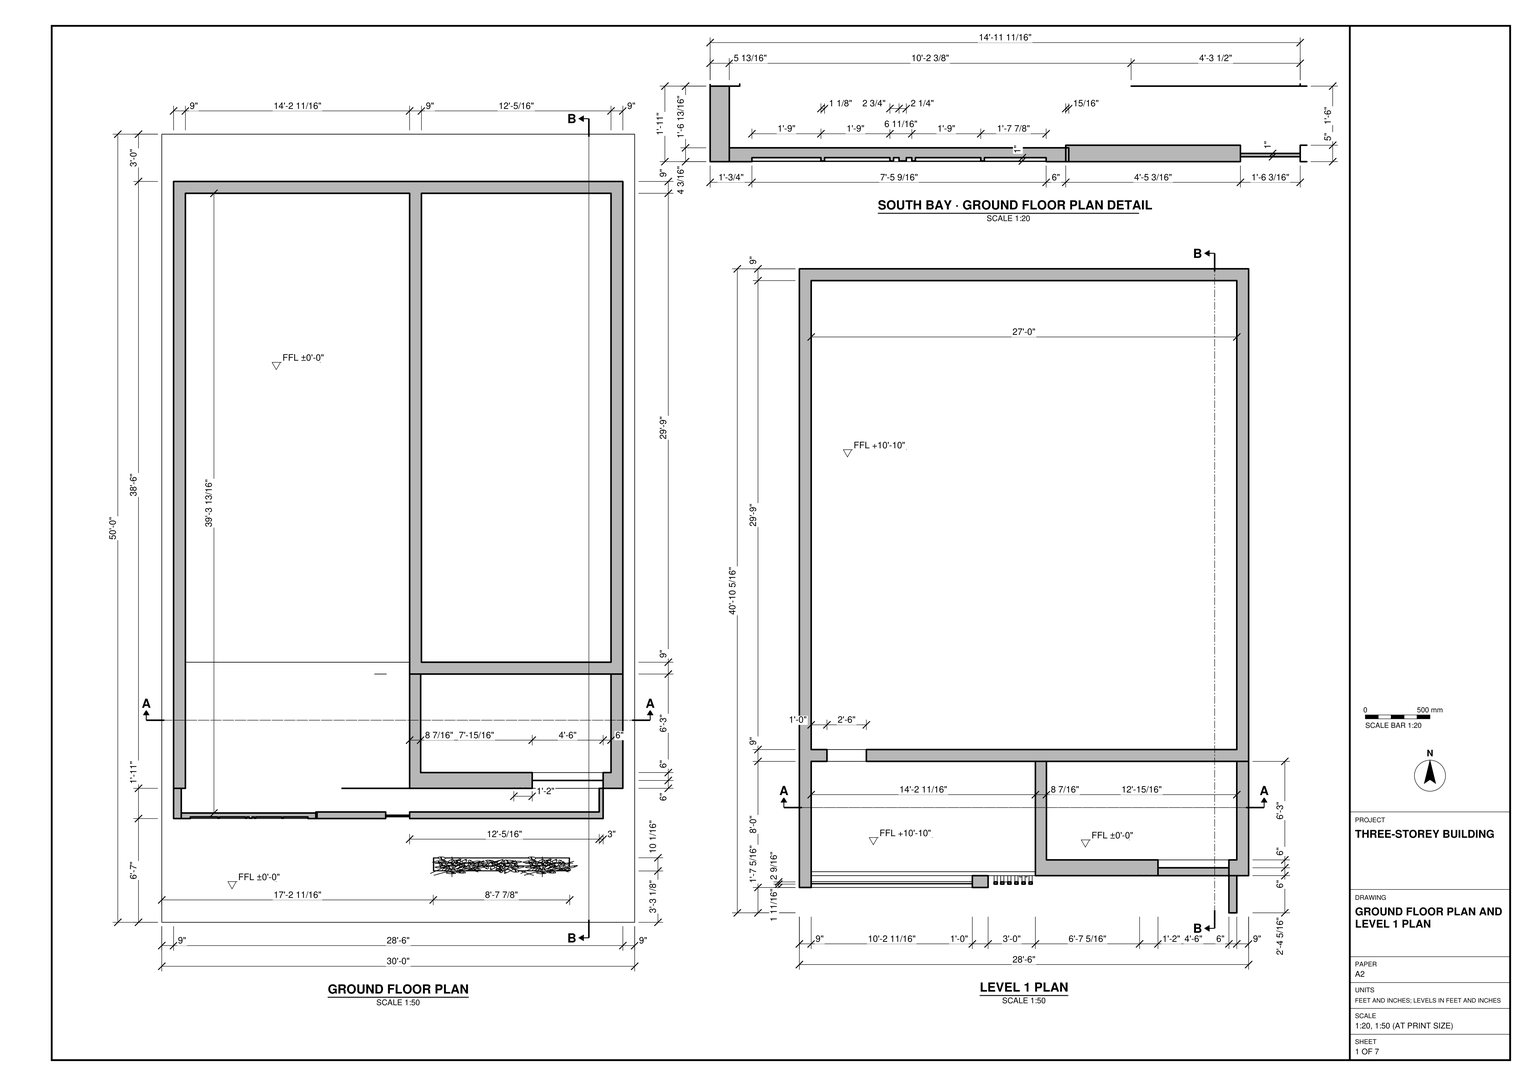
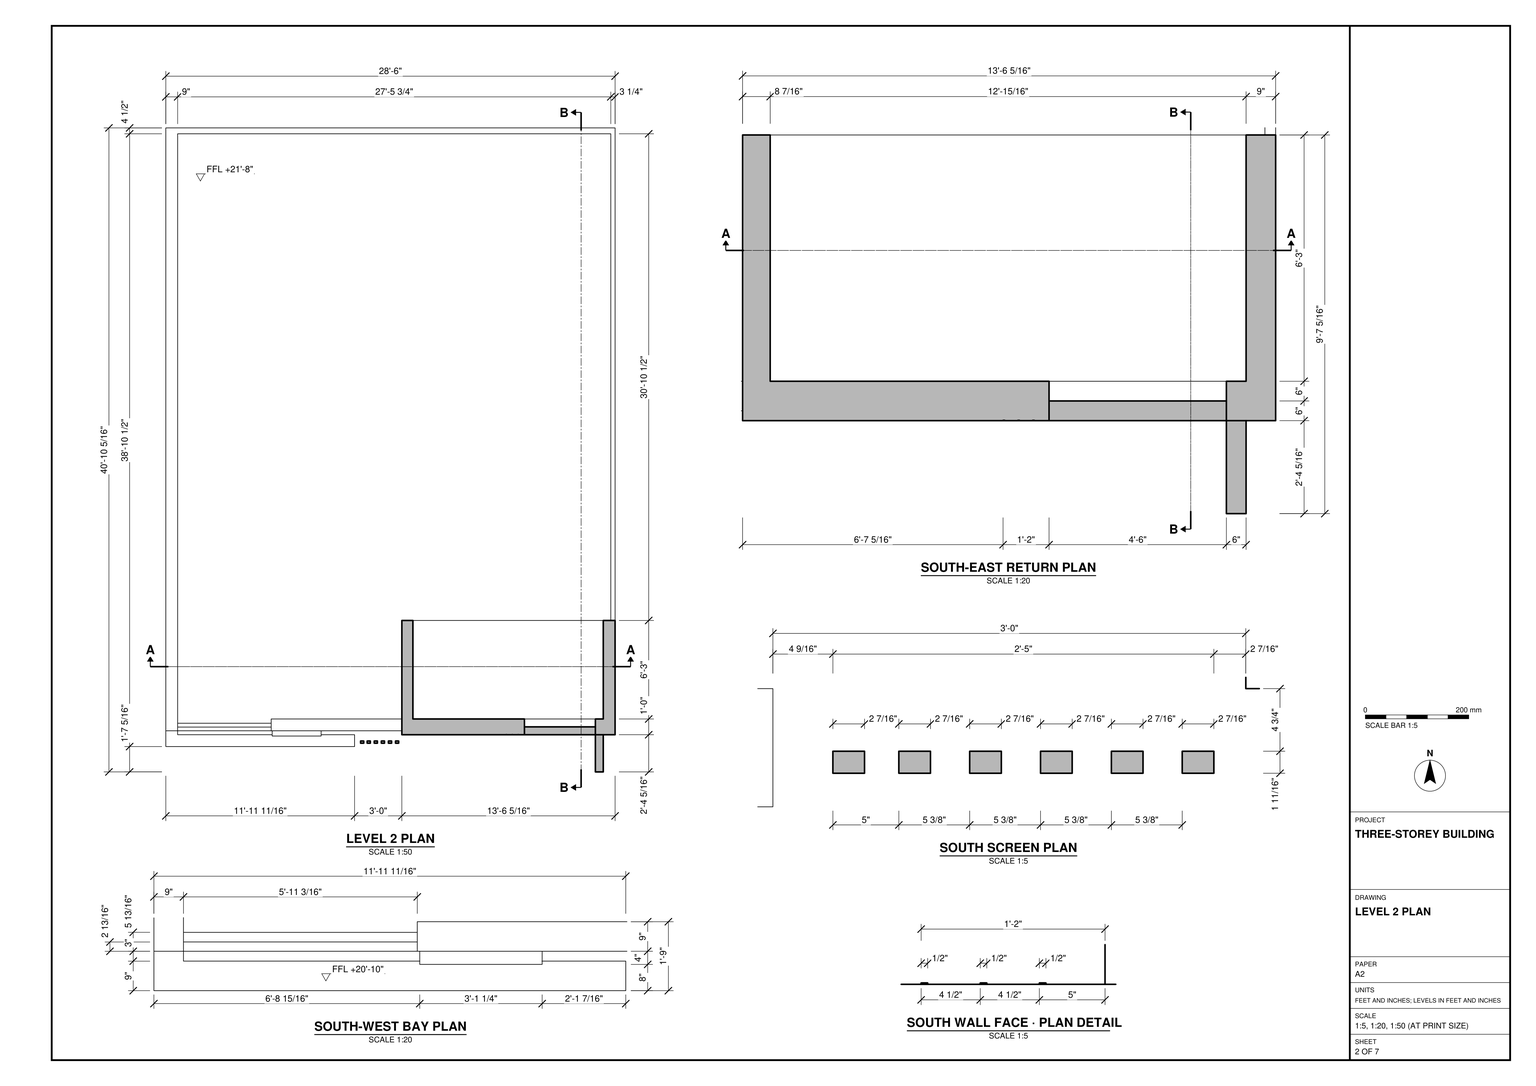
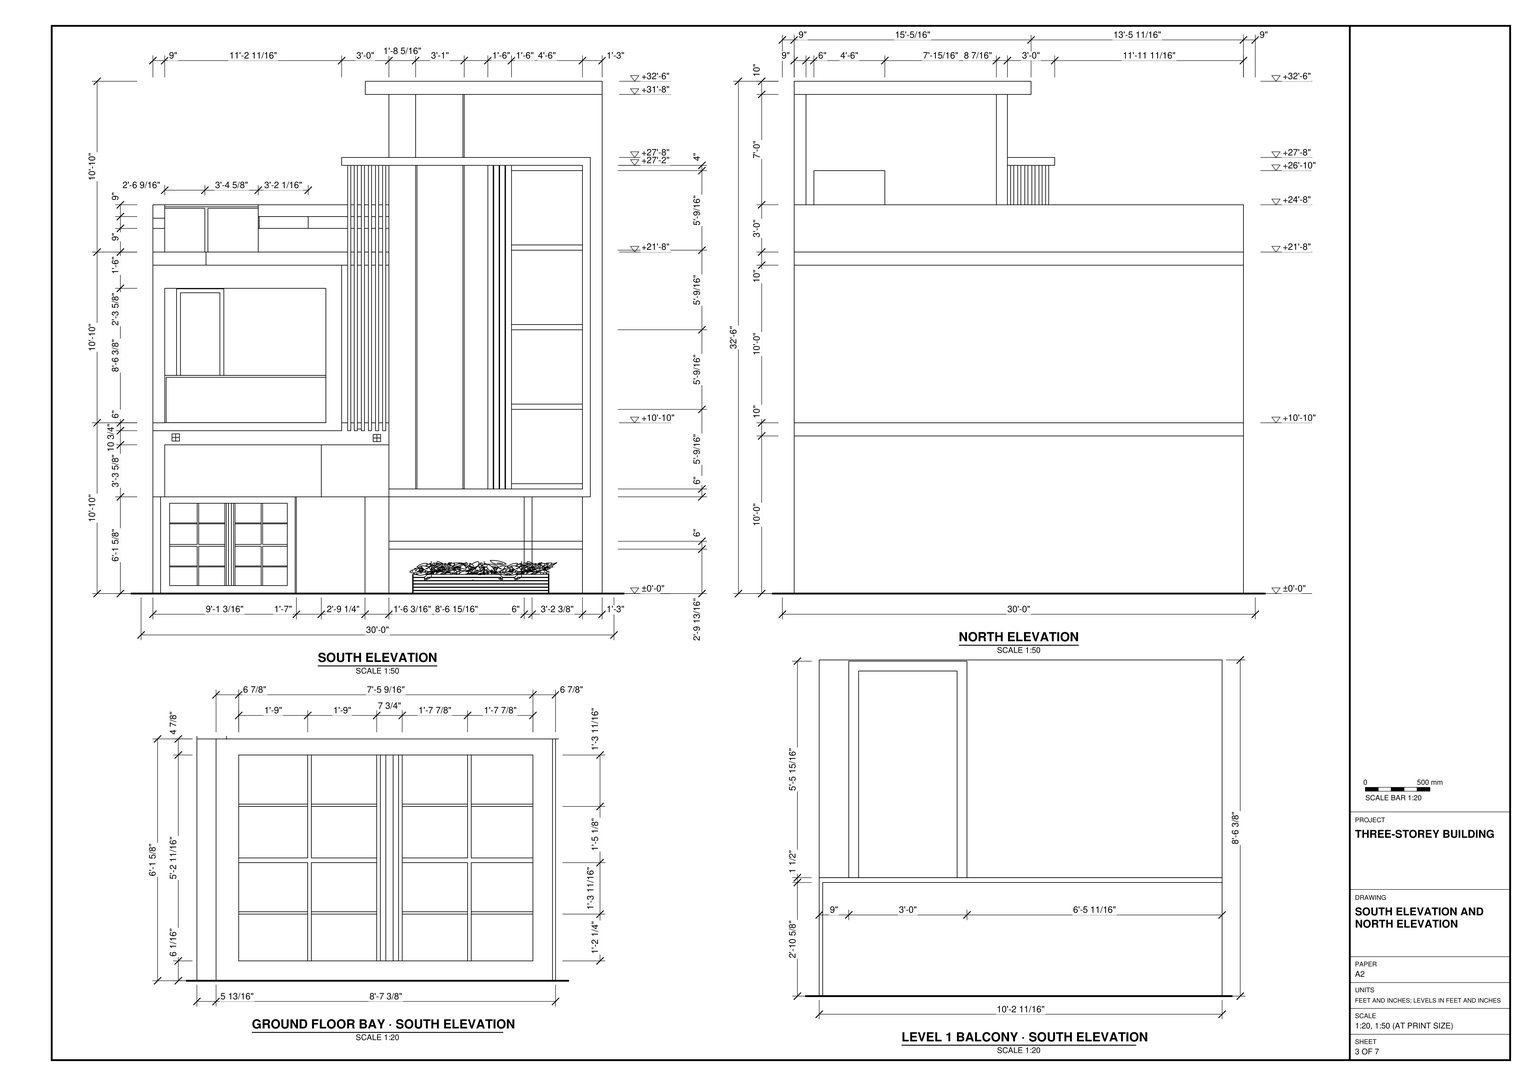
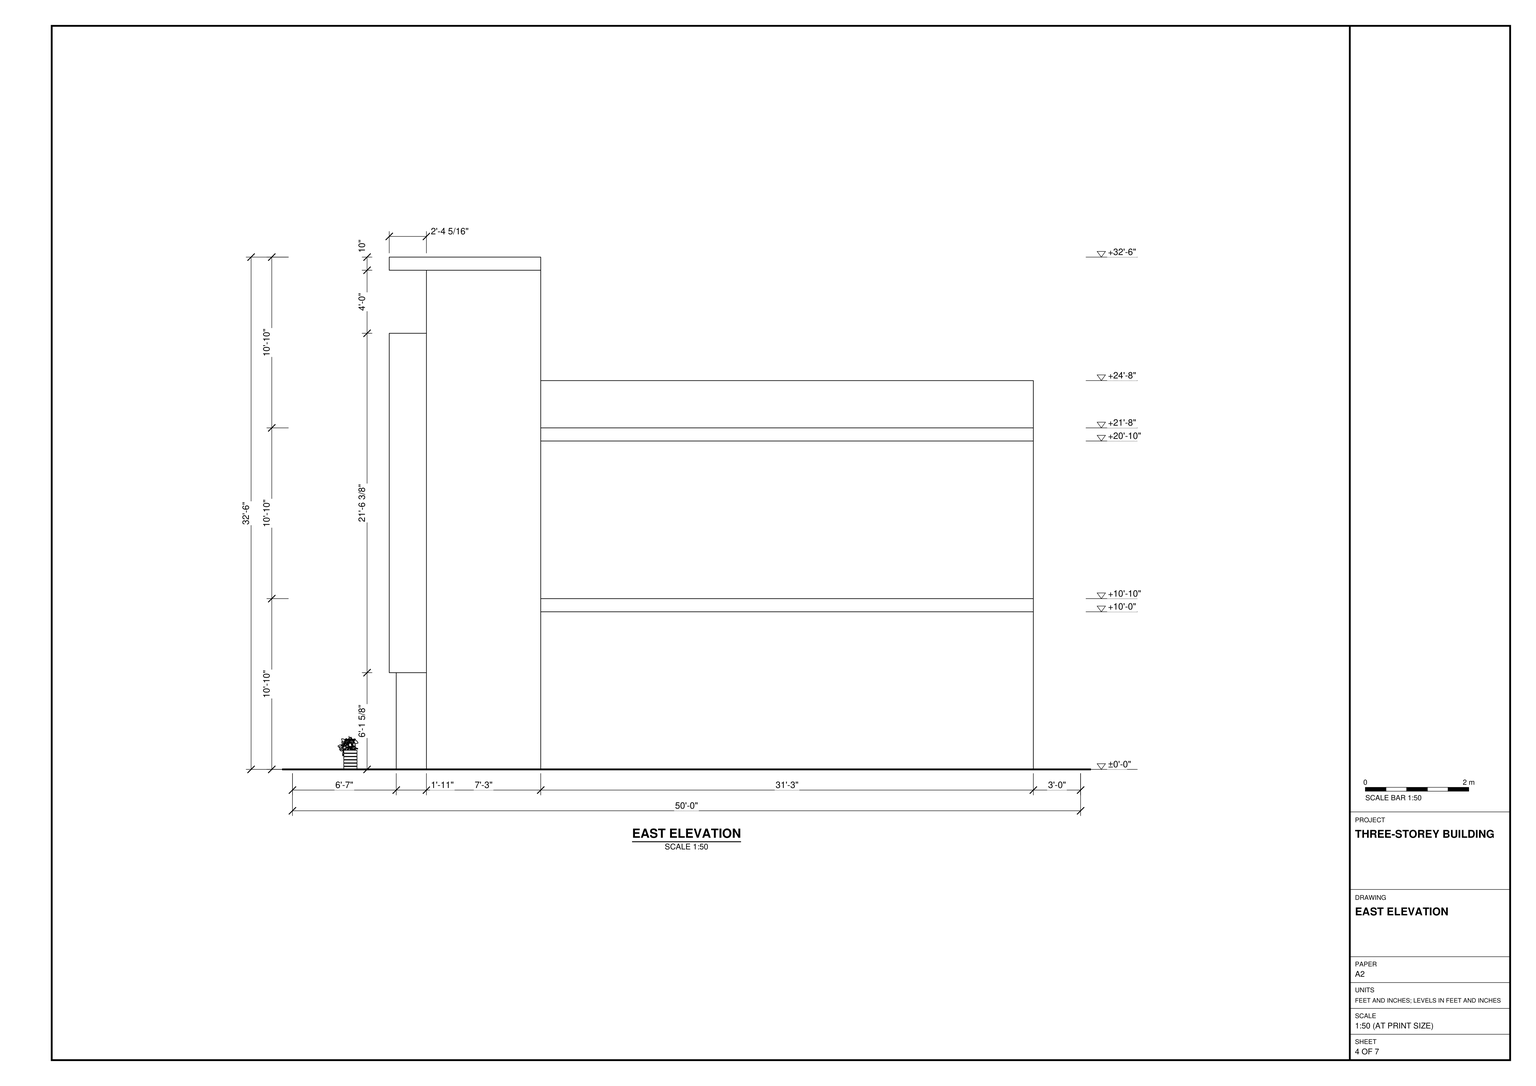
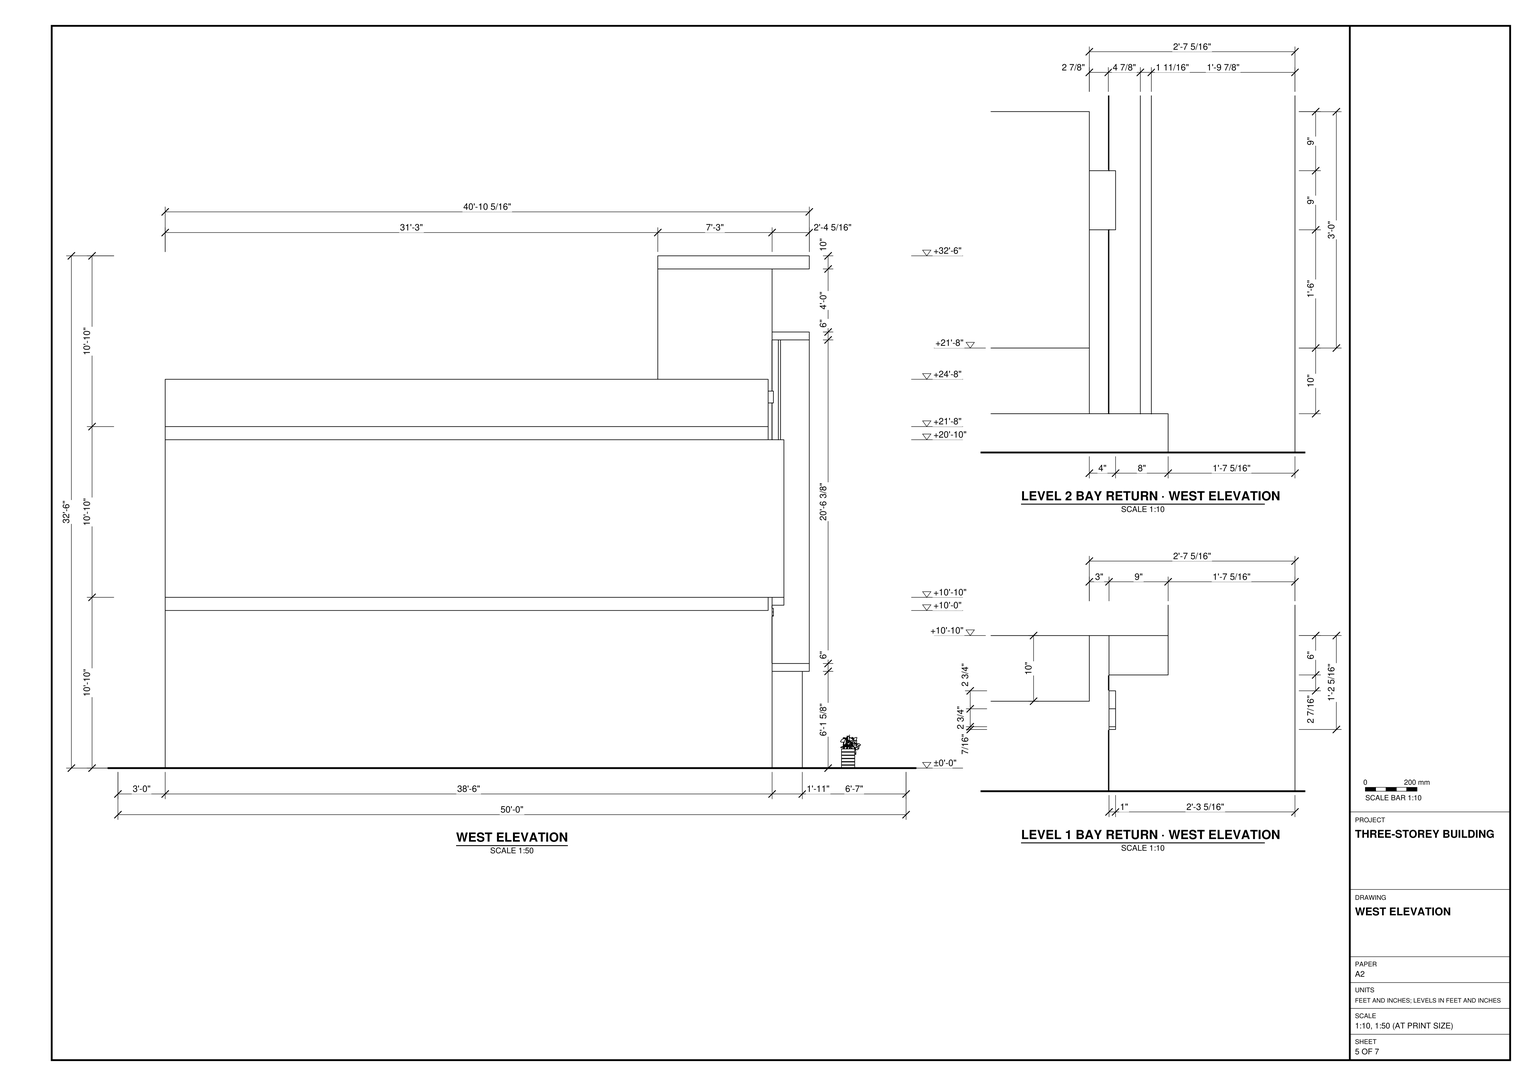
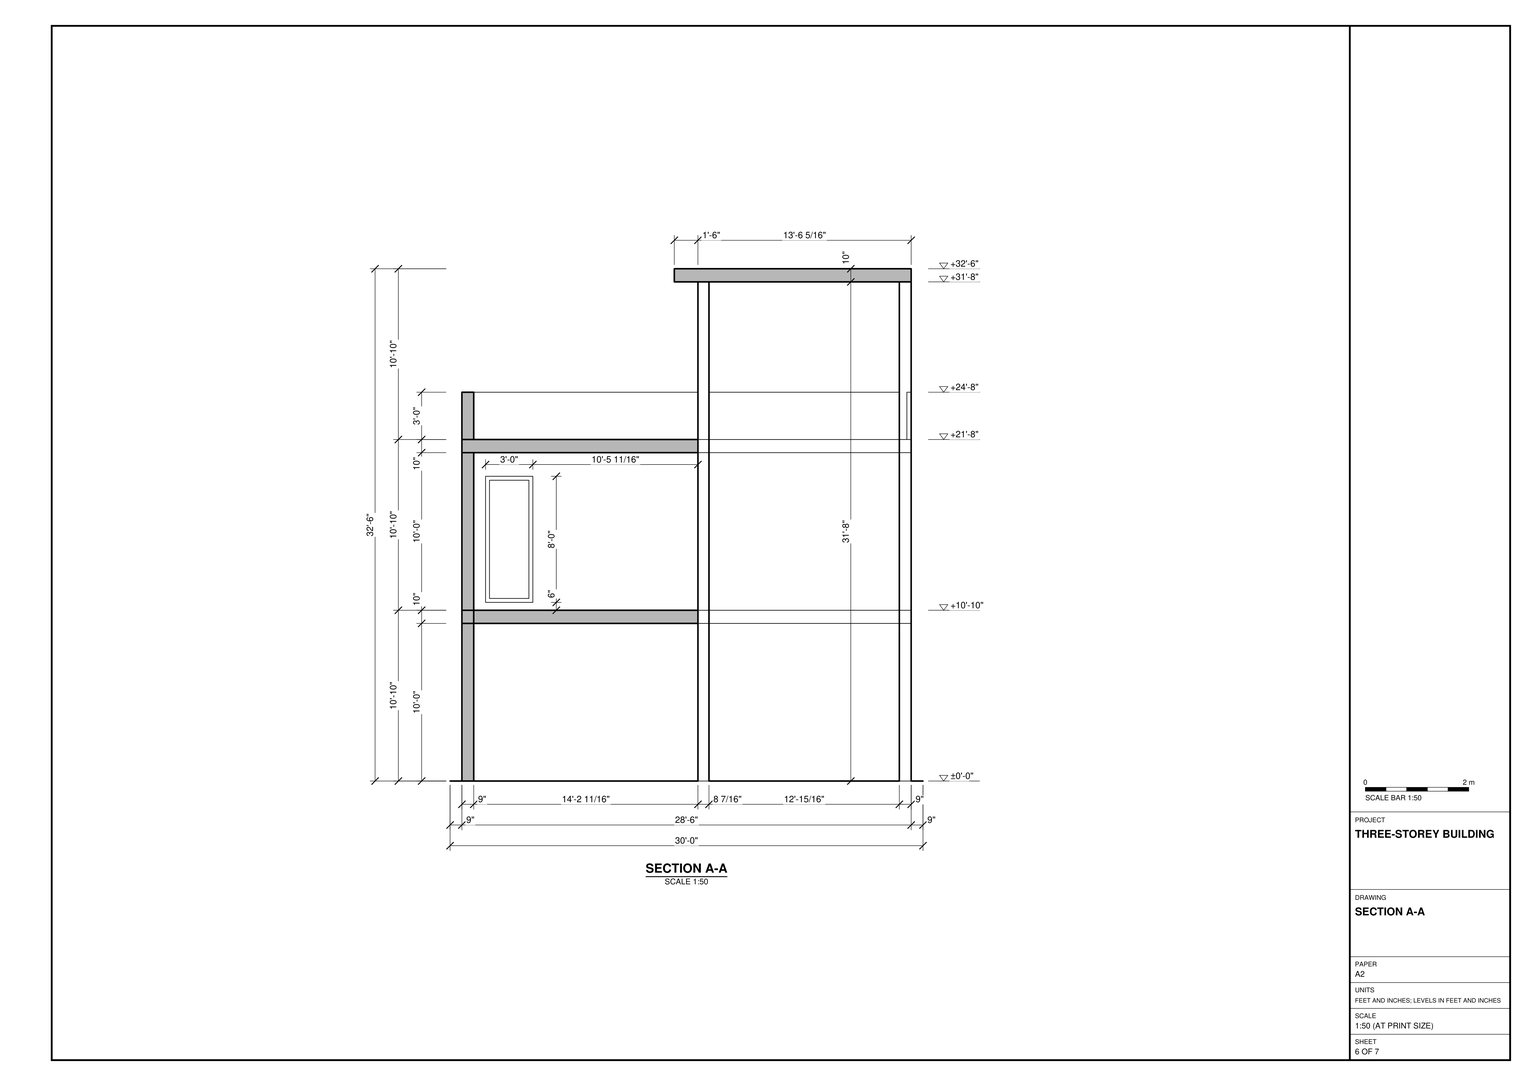
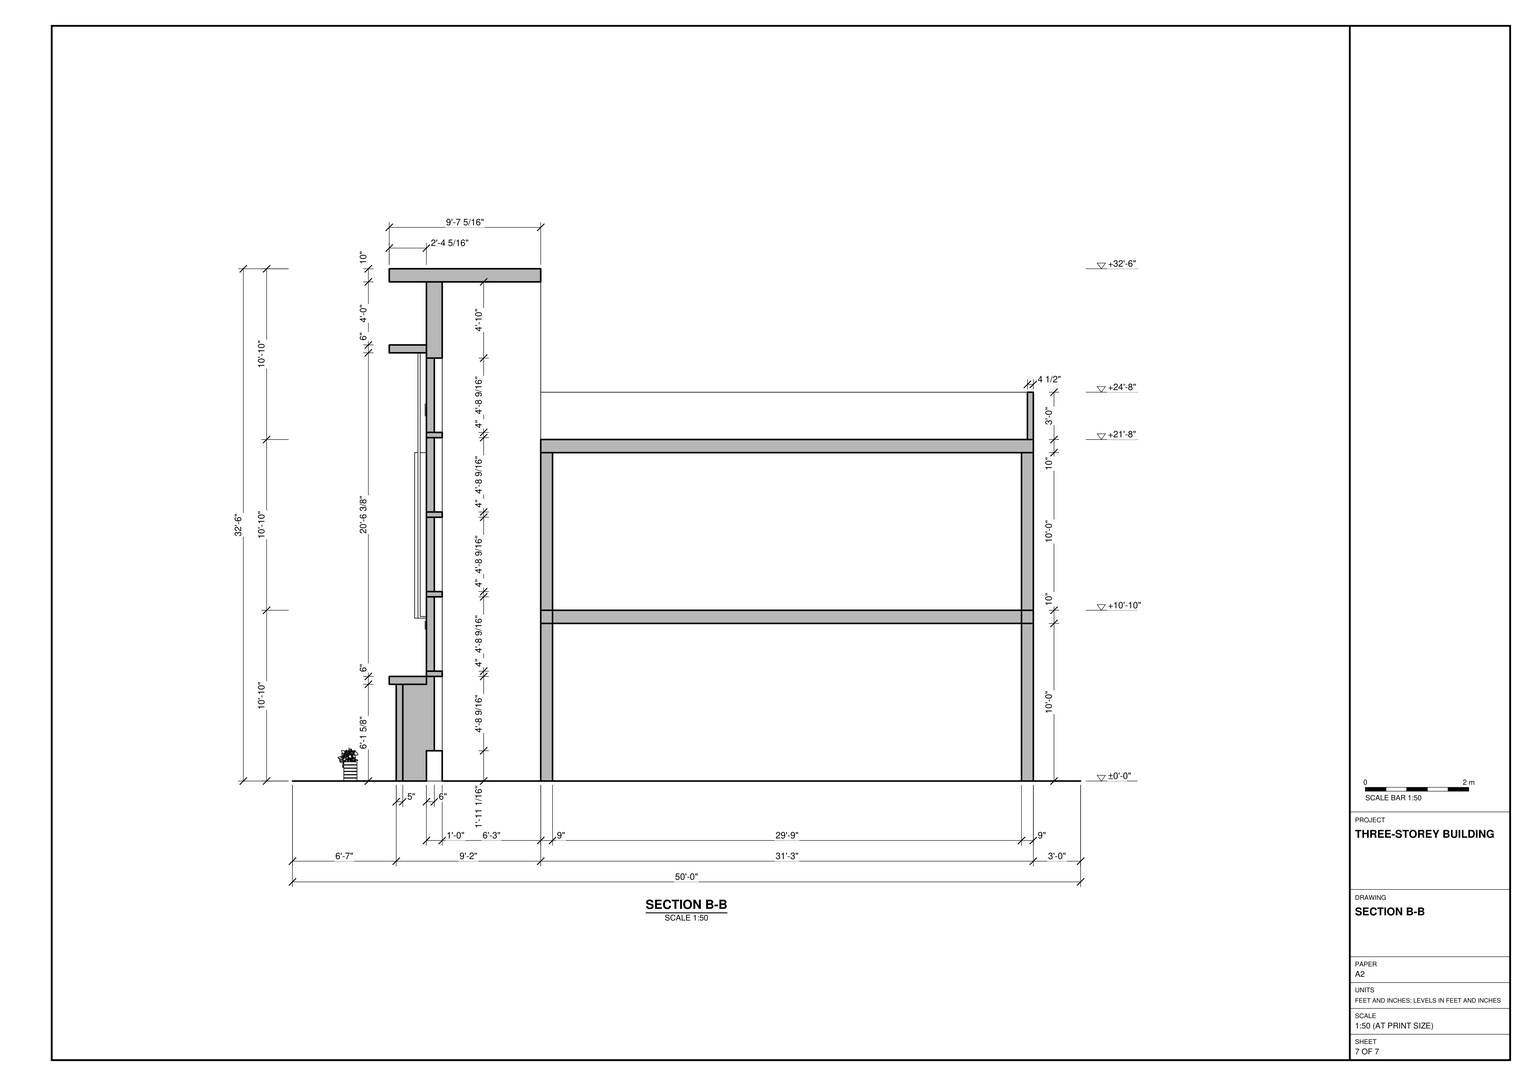
Use task_files/diagram_01.pdf to build the site and three-storey building in SketchUp. Work in feet and inches. The overall model measures 30'-0" across the south frontage, 50'-0" from south to north and 32'-6" high. Set the finished floor levels at ±0'-0", +10'-10" and +21'-8".

Place the building within the site boundary using the setbacks on the ground floor plan. Follow the wall thicknesses shown, including the 9" perimeter walls. On the ground floor, separate the long west space from the east side and place the transverse wall where the rear east space ends. Model the floor slabs, openings and roof edges using the plans and elevations together.

Use the south elevation details for the divided ground floor window bay and the recessed balcony above it. Include the balcony front, the framed opening behind it, the narrow vertical screen beside it and the taller framed bay to the east. Follow the upper plan for the return walls and the flat roof over the raised south-east portion. Place the planted strip in front of the east bay. Plants and other loose decorative items may be suitable library components, for example from 3D Warehouse.

Keep shell elements such as walls, slabs and roof, and each furniture or joinery piece shown, in separate groups or components. Use components for repeated parts. Save one SketchUp model as output_files/three_storey_building_with_screened_south_facade.skp.

# SketchUp Ruby script. Lengths in inches.
U = 1.inch
M = Sketchup.active_model
def pt(a) = Geom::Point3d.new(a.map { |v| v * U })
def face(e, loops, mat)
  f = e.add_face(loops[0].map { |a| pt(a) })
  loops[1..].each { |l| e.add_face(l.map { |a| pt(a) }).erase! }
  f.material = f.back_material = mat if mat
  f
end
# faces: each face lists its corners as indices into pts; further lists are holes
def faces(e, pts, list, mat = nil) = list.each { |f| face(e, (f[0].is_a?(Array) ? f : [f]).map { |l| l.map { |i| pts[i] } }, mat) }
# xy, xz, yz: faces in a plane at the given z, y or x. An outline is a flat list of corners, or four numbers for a rectangle; further outlines are holes
def ring(l) = l.size == 4 ? [[l[0], l[1]], [l[2], l[1]], [l[2], l[3]], [l[0], l[3]]] : l.each_slice(2).to_a
def flat(e, list, mat, &to3) = list.each { |f| face(e, (f[0].is_a?(Array) ? f : [f]).map { |l| ring(l).map { |u, v| to3.(u, v) } }, mat) }
def xy(e, z, list, mat = nil) = flat(e, list, mat) { |x, y| [x, y, z] }
def xz(e, y, list, mat = nil) = flat(e, list, mat) { |x, z| [x, y, z] }
def yz(e, x, list, mat = nil) = flat(e, list, mat) { |y, z| [x, y, z] }
def lines(e, pts, list) = list.each { |a, b| e.add_line(pt(pts[a]), pt(pts[b])) }
# prism: a flat outline (further loops are holes) pulled along v
def prism(e, loops, v, mat = nil)
  f = face(e, loops, mat); d = Geom::Vector3d.new(v.map { |x| x * U })
  f.pushpull(f.normal.samedirection?(d) ? d.length : -d.length)
end
def box(e, o, s, mat = nil) = prism(e, [[o, [o[0] + s[0], o[1], o[2]], [o[0] + s[0], o[1] + s[1], o[2]], [o[0], o[1] + s[1], o[2]]]], [0, 0, s[2]], mat)
def at(x, y, z, deg = 0) = Geom::Transformation.translation(pt([x, y, z])) * Geom::Transformation.rotation(ORIGIN, Z_AXIS, deg.degrees)
def axes(o, x, y, z) = Geom::Transformation.new([*x, 0, *y, 0, *z, 0, *pt(o).to_a, 1])
def part(name) = M.definitions.add(name)
# library, detail: a bought-in or finely detailed component or shape, given as its bounding box
def library(name, o, s) = part(name).tap { |d| box(d.entities, o, s) }
def detail(e, o, s) = box(e.add_group.entities, o, s)
def put(e, d, t, mat = nil) = e.add_instance(d, t).tap { |i| i.material = mat if mat }
def group(e, t, mat = nil) = e.add_group.tap { |g| g.transformation = t; g.material = mat if mat }.entities
root = M.entities
M.materials.add("F01_Seafoam_Drift").color = [229, 255, 204]
M.materials.add("Glass_Basic_01").color = [161, 173, 186]
M.materials["Glass_Basic_01"].alpha = 0.25
M.materials.add("Glass_Mirror_1").color = [162, 156, 185]
M.materials.add("Glass_Safety_01").color = [204, 235, 244]
M.materials["Glass_Safety_01"].alpha = 0.25
M.materials.add("M06_Steel_Smoke").color = [86, 86, 86]
M.materials.add("Wood_Floor_01_1K").color = [146, 111, 76]
M.materials.add("Wood_Floor_12_1K").color = [92, 75, 65]
M.materials.add("Wood_Planks_01_1K").color = [69, 67, 63]
M.materials.add("Wood_Veneer_15_1K").color = [103, 69, 45]
c1 = library("Shrub planter",[0,0,0],[56.02,15.3,25.28])
xy(root,0,[[[0,0,360,600],[188.68,79,188.68,84,333,84,333,102,188.68,102,188.68,189,197.09,189,197.09,114,342,114,342,189,351,189,351,102,336,102,336,79],[117.29,79,170.48,84],[9,79,14.84,102]],[188.68,79,336,79,336,102,333,102,333,84,188.68,84]])
xy(root,18.36,[[272.5,102,273,102.11],[277,102,277.5,102.11]])
xy(root,23.05,[[282,102,336,108],[282,108,336,114]])
xy(root,73.64,[[188.68,73.6875,333,79],[333,73.6875,336,79],[336,73.6875,342,102],[9,79,14.84,102],[117.29,79,170.48,84],
  [188.68,79,333,84],[333,79,336,102],[170.48,80.5,188.68,81.5],[188.68,84,333,102]])
xy(root,79.64,[[188.68,73.6875,336,102],[282,102,336,108],[282,108,336,114]])
xy(root,83.64,[[282,108,336,114]])
xy(root,83.64,[[282,102,336,108]],"Wood_Planks_01_1K")
xy(root,115.7,[[176.7,101,179.53,102],[179.53,101,182.36,102]])
xy(root,116.12,[[23.54,101,26.37,102],[26.37,101,29.2,102]])
xy(root,121.17,[[176.7,101,179.53,102],[179.53,101,182.36,102]])
xy(root,124,[[157.25,95.56,159.66,102],[162.27,95.56,164.68,102],[167.66,95.56,170.07,102],[178.45,95.56,180.86,102],[183.84,95.56,186.25,102]])
xy(root,124,[[173.05,95.56,175.46,102]],"Wood_Veneer_15_1K")
xy(root,125.25,[[157.25,97.23,159.66,102],[162.27,97.23,164.68,102],[167.66,97.23,170.07,102],[178.45,97.23,180.86,102],[183.84,97.23,186.25,102]])
xy(root,125.25,[[173.05,97.23,175.46,102]],"Wood_Veneer_15_1K")
xy(root,140.23,[[282,108,336,114]])
xy(root,140.23,[[282,102,336,108]],"Wood_Planks_01_1K")
xy(root,144.23,[[282,108,336,114]])
xy(root,144.23,[[282,102,336,108]],"Wood_Planks_01_1K")
xy(root,164.6,[[19.07,96.125,140.83,97.42]])
xy(root,200.82,[[282,108,336,114]])
xy(root,200.82,[[282,102,336,108]],"Wood_Planks_01_1K")
xy(root,204.82,[[282,108,336,114]])
xy(root,204.82,[[282,102,336,108]],"Wood_Planks_01_1K")
xy(root,258.92,[[48.56,107.83,50.87,110.75]])
xy(root,260,[[9,105,9,564,351,564,351,189,347.73,189,347.73,559.5,18,559.5,18,105],[89.19,105,188.68,114]])
xy(root,261.41,[[282,108,336,114]])
xy(root,261.41,[[282,102,336,108]],"Wood_Planks_01_1K")
xy(root,265.41,[[282,108,336,114]])
xy(root,265.41,[[282,102,336,108]],"Wood_Planks_01_1K")
xy(root,278,[[89.95,101,127.22,105],[127.22,105,188.68,114]])
xy(root,287,[[89.95,101,127.22,105],[127.22,105,188.68,114]])
xy(root,293.29,[[18,107.83,48.56,109.29],[50.87,107.83,89.19,109.29],[18,109.29,48.56,110.75],[50.87,109.29,89.19,110.75]])
xy(root,294.45,[[18,107.83,89.19,110.75]])
xy(root,296,[[9,105,18,105,18,559.5,347.73,559.5,347.73,189,351,189,351,564,9,564],[89.19,105,188.68,114]])
xy(root,322,[[282,108,336,114]])
xy(root,322,[[282,102,336,108]],"Wood_Planks_01_1K")
xy(root,326,[[[152.68,73.6875,152.68,102,268,102,268,102.11,268.5,102.11,268.5,102,272.5,102,272.5,102.11,273,102.11,273,102,277,102,277,102.11,277.5,102.11,277.5,102,336,102,336,73.6875],[157.25,95.56,159.66,97.23]]])
xy(root,332,[[152.68,73.6875,342,102]])
xy(root,380,[[170.68,73.6875,170.68,189,188.68,189,188.68,102,351,102,351,73.6875],[188.68,102,351,114],[188.68,114,197.09,189],[197.09,114,342,189],[342,114,351,189]])
xy(root,390,[[170.68,73.6875,351,189]])
xz(root,73.6875,[[170.68,380,351,390]])
xz(root,73.6875,[[188.68,73.64,342,73.64,342,332,152.68,332,152.68,326,336,326,336,79.64,188.68,79.64]],"M06_Steel_Smoke")
xz(root,79,[[291.64,0,297.64,33.82],[188.68,33.82,291.64,39.82],[291.64,33.82,297.64,39.82],[297.64,33.82,336,39.82],[291.64,39.82,297.64,73.64]])
xz(root,79,[[117.29,0,170.48,73.64],[188.68,0,291.64,33.82],[297.64,0,336,33.82],[188.68,39.82,291.64,73.64],[297.64,39.82,336,73.64]],"F01_Seafoam_Drift")
xz(root,79,[[9,0,14.84,73.64]],"Wood_Planks_01_1K")
xz(root,80.5,[[170.48,0,188.68,73.64]],"Wood_Floor_01_1K")
xz(root,81.5,[[170.48,0,188.68,73.64]])
xz(root,84,[[117.29,0,170.48,73.64],[188.68,0,333,73.64]])
xz(root,95.56,[[157.25,124,159.66,326],[162.27,124,164.68,326],[167.66,124,170.07,326],[173.05,124,175.46,326],[178.45,124,180.86,326],
  [183.84,124,186.25,326]],"Wood_Veneer_15_1K")
xz(root,97.23,[[157.25,125.25,159.66,326],[162.27,125.25,164.68,326],[167.66,125.25,170.07,326],[178.45,125.25,180.86,326],[183.84,125.25,186.25,326]])
xz(root,97.23,[[173.05,125.25,175.46,326]],"Wood_Veneer_15_1K")
xz(root,101,[[176.7,115.7,179.53,118.43],[179.53,115.7,182.36,118.43],[23.54,116.12,26.37,118.85],[26.37,116.12,29.2,118.85],[176.7,118.43,179.53,121.17],
  [179.53,118.43,182.36,121.17],[23.54,118.85,26.37,121.59],[26.37,118.85,29.2,121.59],[89.95,278,127.22,287]])
xz(root,102,[[9,0,14.84,73.64],[188.68,0,209,73.64],[209,0,210.01,73.64],[210.01,0,245,73.64],[245,0,246,73.64],
  [246,0,264,73.64],[264,0,333,0,333,19.05,282,19.05,282,18.36,268.5,18.36,268,18.37,264,18.37],[333,0,336,19.05],[268.5,18.36,272.5,73.64],[273,18.36,277,73.64],
  [277.5,18.36,282,73.64],[264,18.37,268,73.64],[282,19.05,333,23.05],[333,19.05,336,23.05],[333,23.05,336,73.64],
  [188.68,73.64,209,79.64],[209,73.64,210.01,79.64],[210.01,73.64,245,79.64],[245,73.64,246,79.64],[246,73.64,264,79.64],
  [264,73.64,268,79.64],[268,73.64,268.5,79.64],[268.5,73.64,272.5,79.64],[272.5,73.64,273,79.64],[273,73.64,277,79.64],
  [277,73.64,277.5,79.64],[277.5,73.64,282,79.64],[282,73.64,336,79.64],[209,79.64,210.01,326],[245,79.64,246,326],
  [157.25,124,159.66,125.25],[162.27,124,164.68,125.25],[167.66,124,170.07,125.25],[178.45,124,180.86,125.25],[183.84,124,186.25,125.25],
  [152.68,326,188.68,332],[188.68,326,209,332],[209,326,245,332]])
xz(root,102,[[336,0,351,0,351,380,246,380,246,332,342,332,342,73.64,336,73.64],[188.68,79.64,209,326],[210.01,79.64,245,326],[246,79.64,264,326],[188.68,332,209,380],
  [209,332,245,380],[245,332,246,380]],"F01_Seafoam_Drift")
xz(root,102,[[336,73.64,342,73.64,342,332,245,332,245,326,268,326,268,79.64,268.5,79.64,268.5,326,272.5,326,272.5,79.64,273,79.64,273,326,277,326,277,79.64,277.5,79.64,277.5,326,336,326,336,322,282,322,282,265.41,336,265.41,336,261.41,282,261.41,282,204.82,336,204.82,336,200.82,282,200.82,282,144.23,336,144.23,336,140.23,282,140.23,282,83.64,336,83.64]],"Glass_Mirror_1")
xz(root,102,[[137.2,0,188.68,113.24]],"Wood_Floor_01_1K")
xz(root,102,[[282,79.64,336,83.64],[282,140.23,336,144.23],[282,200.82,336,204.82],[282,261.41,336,265.41],[282,322,336,326]],"Wood_Planks_01_1K")
xz(root,102,[[264,79.64,268,326],[268.5,79.64,272.5,326],[273,79.64,277,326],[277.5,79.64,282,326],[173.05,124,175.46,125.25]],"Wood_Veneer_15_1K")
xz(root,102.11,[[268.5,18.36,268.5,326,268,326,268,18.37],[272.5,18.36,273,326],[277,18.36,277.5,326]])
xz(root,105,[[9,278,18,285.73],[89.19,278,89.95,287],[89.95,278,127.22,287]])
xz(root,105,[[9,260,18,278],[89.19,260,188.68,278],[9,285.73,18,296],[89.19,287,188.68,296]],"M06_Steel_Smoke")
xz(root,107.83,[[48.56,258.92,50.87,258.92,50.87,293.29,89.19,293.29,89.19,294.45,18,294.45,18,293.29,48.56,293.29]])
xz(root,108,[[282,23.05,336,79.64]])
xz(root,108,[[282,144.23,336,200.82],[282,204.82,336,261.41],[282,265.41,336,322]],"Glass_Basic_01")
xz(root,108,[[282,83.64,336,140.23]],"Glass_Safety_01")
xz(root,109.29,[[18,260,48.56,293.29],[50.87,260,89.19,293.29]],"Glass_Safety_01")
xz(root,110.75,[[48.56,258.92,48.56,293.29,18,293.29,18,294.45,89.19,294.45,89.19,293.29,50.87,293.29,50.87,258.92]])
xz(root,114,[[[197.09,0,342,380],[282,265.41,336,322],[282,144.23,336,200.82],[282,83.64,336,140.23],[282,204.82,336,261.41],[282,23.05,336,79.64]],[89.19,260,89.19,296,188.68,296,188.68,287,127.22,287,127.22,278,188.68,278,188.68,260]])
xz(root,189,[[188.68,0,197.09,380],[342,0,342,380,351,380,351,296,347.73,296,347.73,260,351,260,351,0],[170.68,380,351,390]])
xz(root,559.5,[[18,260,347.73,296]])
xz(root,564,[[9,260,351,296]])
yz(root,9,[[79,0,102,73.64],[105,260,564,296]])
yz(root,14.84,[[79,0,102,73.64]])
yz(root,18,[[96.875,130.08,95.59,130.1,96.15,166.1,97.4375,166.08],[105,260,109.29,260,109.29,293.29,107.83,293.29,107.83,294.45,110.75,294.45,110.75,293.29,109.29,293.29,109.29,260,559.5,260,559.5,296,105,296]])
yz(root,19.07,[[96.875,130.08,97.42,164.6,96.125,164.6,96.1,163.1,95.59,130.1]])
yz(root,23.54,[[101,116.12,102,118.85],[101,118.85,102,121.59]])
yz(root,29.2,[[101,116.12,102,118.85],[101,118.85,102,121.59]])
yz(root,48.56,[[107.83,258.92,110.75,293.29]])
yz(root,50.87,[[107.83,258.92,110.75,293.29]])
yz(root,89.19,[[105,260,105,296,114,296,114,260,109.29,260,109.29,293.29,110.75,293.29,110.75,294.45,107.83,294.45,107.83,293.29,109.29,293.29,109.29,260]])
yz(root,89.95,[[101,278,105,287]])
yz(root,117.29,[[79,0,84,73.64]])
yz(root,127.22,[[101,278,105,287],[105,278,114,287]])
yz(root,140.83,[[96.125,164.6,97.42,164.6,97.4375,166.08,96.15,166.1]])
yz(root,152.68,[[73.6875,326,102,332]])
yz(root,157.25,[[95.56,124,95.56,326,97.23,326,97.23,125.25,102,125.25,102,124]])
yz(root,159.66,[[95.56,124,102,124,102,125.25,97.23,125.25,97.23,326,95.56,326]])
yz(root,162.27,[[95.56,124,95.56,326,97.23,326,97.23,125.25,102,125.25,102,124]])
yz(root,164.68,[[95.56,124,102,124,102,125.25,97.23,125.25,97.23,326,95.56,326]])
yz(root,167.66,[[95.56,124,95.56,326,97.23,326,97.23,125.25,102,125.25,102,124]])
yz(root,170.07,[[95.56,124,102,124,102,125.25,97.23,125.25,97.23,326,95.56,326]])
yz(root,170.48,[[79,0,80.5,73.64],[80.5,0,84,73.64]])
yz(root,170.68,[[73.6875,380,189,390]])
yz(root,173.05,[[95.56,124,95.56,326,97.23,326,97.23,125.25,102,125.25,102,124]],"Wood_Veneer_15_1K")
yz(root,175.46,[[95.56,124,102,124,102,125.25,97.23,125.25,97.23,326,95.56,326]],"Wood_Veneer_15_1K")
yz(root,176.7,[[101,115.7,102,118.43],[101,118.43,102,121.17]])
yz(root,178.45,[[95.56,124,95.56,326,97.23,326,97.23,125.25,102,125.25,102,124]])
yz(root,180.86,[[95.56,124,102,124,102,125.25,97.23,125.25,97.23,326,95.56,326]])
yz(root,182.36,[[101,115.7,102,118.43],[101,118.43,102,121.17]])
yz(root,183.84,[[95.56,124,95.56,326,97.23,326,97.23,125.25,102,125.25,102,124]])
yz(root,186.25,[[95.56,124,102,124,102,125.25,97.23,125.25,97.23,326,95.56,326]])
yz(root,188.68,[[79,0,80.5,33.82],[80.5,0,84,33.82],[[102,0,189,380],[105,260,114,278],[105,287,114,296]],[79,33.82,80.5,39.82],[80.5,33.82,84,39.82],
  [79,39.82,80.5,73.64],[80.5,39.82,84,73.64],[73.6875,73.64,102,79.64],[105,260,114,278],[105,287,114,296]])
yz(root,197.09,[[114,0,189,380]])
yz(root,268,[[102,18.37,102.11,326]])
yz(root,268.5,[[102,18.36,102.11,326]])
yz(root,272.5,[[102,18.36,102.11,326]])
yz(root,273,[[102,18.36,102.11,326]])
yz(root,277,[[102,18.36,102.11,326]])
yz(root,277.5,[[102,18.36,102.11,326]])
yz(root,282,[[102,23.05,108,79.64],[108,23.05,114,79.64],[108,83.64,114,140.23],[108,144.23,114,200.82],[108,204.82,114,261.41],
  [108,265.41,114,322]])
yz(root,282,[[102,83.64,108,140.23],[102,144.23,108,200.82],[102,204.82,108,261.41],[102,265.41,108,322]],"Wood_Planks_01_1K")
yz(root,333,[[84,0,102,73.64]])
yz(root,336,[[102,23.05,102,79.64,73.6875,79.64,73.6875,326,102,326,102,322,108,322,108,265.41,102,265.41,102,261.41,108,261.41,108,204.82,102,204.82,102,200.82,108,200.82,108,144.23,102,144.23,102,140.23,108,140.23,108,83.64,102,83.64,102,79.64,108,79.64,108,23.05],[108,23.05,114,68.44],[108,68.44,114,79.64],[108,83.64,114,140.23],[108,144.23,114,200.82],
  [108,204.82,114,261.41],[108,265.41,114,322]])
yz(root,336,[[79,0,102,73.64]],"F01_Seafoam_Drift")
yz(root,342,[[114,0,189,380]])
yz(root,342,[[73.6875,73.64,102,332]],"F01_Seafoam_Drift")
yz(root,347.73,[[189,260,559.5,296]])
yz(root,351,[[73.6875,380,189,390]])
yz(root,351,[[102,0,189,380],[189,260,564,296]],"F01_Seafoam_Drift")
p = [[268,102,18.37],[268.5,102,18.36],[268.5,102.11,18.36],[268,102.11,18.37],[19.07,96.875,130.08],[19.07,95.59,130.1],
  [18,95.59,130.1],[18,96.875,130.08],[19.07,96.1,163.1],[19.07,96.125,164.6],[140.83,96.125,164.6],[140.83,96.15,166.1],
  [18,96.15,166.1],[140.83,95.59,130.1],[18,97.4375,166.08],[140.83,97.4375,166.08],[140.83,97.42,164.6],[19.07,97.42,164.6],
  [162,189,0],[171,189,0],[167.66,97.23,125.25],[167.59,97.23,125.25],[164.68,97.23,125.25]]
faces(root,p,[[0,1,2,3],[4,5,6,7],[6,5,8,9,10,11,12],[4,7,14,15,16,17],[12,11,15,14]])
faces(root,p,[[10,9,8,5,13]],"Glass_Basic_01")
lines(root,p,[[18,19],[20,21],[21,22]])
put(root,c1,axes([204.5,34.62,0],[2,0,0],[0,1,0],[0,0,1]))
g1 = group(root,at(9,189,0),"F01_Seafoam_Drift")
xy(g1,0,[[0,-87,9,0],[[0,0,9,0,9,366,179.68,366,179.68,0,342,0,342,375,0,375],[188.68,9,333,366]],[9,9,179.68,366],[188.68,9,333,366]])
xy(g1,113.24,[[9,-87,179.68,-84]])
xy(g1,120,[[9,0,179.68,9],[179.68,9,188.68,366]])
xy(g1,130,[[[0,-87,179.68,-87,179.68,-84,9,-84,9,0,342,0,342,375,0,375],[9,9,333,366]]])
xz(g1,-87,[[0,0,9,0,9,113.24,179.68,113.24,179.68,130,0,130]],"Wood_Planks_01_1K")
xz(g1,-84,[[9,113.24,179.68,130]])
xz(g1,0,[[179.68,0,342,0,342,130,9,130,9,120,179.68,120]])
xz(g1,9,[[188.68,0,188.68,120,9,120,9,130,333,130,333,0]])
xz(g1,366,[[9,0,179.68,0,179.68,120,188.68,120,188.68,0,333,0,333,130,9,130]])
xz(g1,375,[[0,0,342,130]])
yz(g1,0,[[-87,0,375,130]])
yz(g1,9,[[-87,0,9,0,9,120,0,120,0,130,-84,130,-84,113.24,-87,113.24],[9,0,366,130]])
yz(g1,179.68,[[0,0,366,120],[-87,113.24,-84,130]])
yz(g1,188.68,[[9,0,366,120]])
yz(g1,333,[[9,0,366,130]])
yz(g1,342,[[0,0,375,130]])
g2 = group(root,at(9,189,250))
xy(g2,0,[[0,-84,0,375,342,375,342,0,179.68,0,179.68,-84]])
xy(g2,10,[[0,-84,179.68,-84,179.68,0,342,0,342,375,0,375]])
xz(g2,-84,[[40.44,0,179.68,10]])
xz(g2,-84,[[0,0,40.44,10]],"M06_Steel_Smoke")
xz(g2,0,[[179.68,0,342,10]])
xz(g2,375,[[0,0,342,10]])
yz(g2,0,[[-84,0,375,10]])
yz(g2,179.68,[[-84,0,0,10]])
yz(g2,342,[[0,0,375,10]])
p = [[39.56,-79.71,10],[39.56,-79.71,9.18],[39.56,-79.71,0]]
lines(g2,p,[[0,1],[1,2]])
g3 = group(root,at(9,189,120))
prism(g3,[[[0,-84,0],[0,375,0],[342,375,0],[342,0,0],[179.68,0,0],[179.68,-84,0]]],[0,0,10])
g4 = group(root,at(9,189,130),"F01_Seafoam_Drift")
xy(g4,-6,[[0,-96,143.68,-87]])
xy(g4,0,[[0,-96,9,-87],[0,-87,9,0],[9,9,333,366]])
xy(g4,9,[[21,0,51,9]])
xy(g4,99,[[21,0,51,9]])
xy(g4,102.375,[[9,-96,131.68,-87]])
xy(g4,120,[[[0,-96,143.68,-96,143.68,-87,9,-87,9,0,342,0,342,375,0,375],[9,9,333,366]]])
xz(g4,-96,[[[0,-6,143.68,120],[9,0.14,131.68,102.375]]])
xz(g4,-87,[[0,-6,0,0,131.68,0,131.68,102.375,9,102.375,9,120,143.68,120,143.68,-6]])
xz(g4,0,[[[18,6,54,102],[21,9,51,99]]])
xz(g4,0,[[[9,0,342,120],[18,6,54,102]]],"Wood_Veneer_15_1K")
xz(g4,9,[[[9,0,333,120],[21,9,51,99]]])
xz(g4,366,[[9,0,333,120]])
xz(g4,375,[[0,0,342,120]])
yz(g4,0,[[-96,-6,-87,0],[-96,0,375,120]])
yz(g4,9,[[-87,0,-87,102.375,-96,102.375,-96,0.14],[-96,0,-96,0.14,-87,0],[-87,0,0,120],[9,0,366,120]])
yz(g4,21,[[0,9,9,99]])
yz(g4,51,[[0,9,9,99]])
yz(g4,131.68,[[-87,0,-96,0.14,-96,102.375,-87,102.375]])
yz(g4,143.68,[[-96,-6,-87,120]])
yz(g4,333,[[9,0,366,120]])
yz(g4,342,[[0,0,375,120]])
p = [[131.68,-96,0.14],[131.68,-87,0],[9,-87,0],[9,-96,0.14]]
faces(g4,p,[[0,1,2,3]])
g5 = group(root,at(14.84,79,0))
xy(g5,0,[[0,0,103.37,4.21]])
xy(g5,6.04,[[6.89,0,48.91,0,48.91,1.21,29.01,1.21,29.01,0.21,27.9,0.21,27.9,1.21,6.89,1.21],[48.91,0,50.02,0.21],[50.02,0,51.68,1.21],[51.68,0,53.9,0.21],[53.9,0,55.57,1.21],
  [55.57,0,56.68,0.21],[56.68,0,96.48,0,96.48,1.21,77.6875,1.21,77.6875,0.21,76.58,0.21,76.58,1.21,56.68,1.21]])
xy(g5,20.29,[[6.89,0.21,27.9,1.21],[29.01,0.21,48.91,1.21],[56.68,0.21,76.58,1.21],[77.6875,0.21,96.48,1.21]])
xy(g5,21.01,[[6.89,0.21,27.9,1.21],[29.01,0.21,48.91,1.21],[56.68,0.21,76.58,1.21],[77.6875,0.21,96.48,1.21]])
xy(g5,35.97,[[6.89,0.21,27.9,1.21],[29.01,0.21,48.91,1.21],[56.68,0.21,76.58,1.21],[77.6875,0.21,96.48,1.21]])
xy(g5,37.4,[[6.89,0.21,27.9,1.21],[29.01,0.21,48.91,1.21],[56.68,0.21,76.58,1.21],[77.6875,0.21,96.48,1.21]])
xy(g5,53.07,[[6.89,0.21,27.9,1.21],[29.01,0.21,48.91,1.21],[56.68,0.21,76.58,1.21],[77.6875,0.21,96.48,1.21]])
xy(g5,53.79,[[6.89,0.21,27.9,1.21],[29.01,0.21,48.91,1.21],[56.68,0.21,76.58,1.21],[77.6875,0.21,96.48,1.21]])
xy(g5,68.75,[[6.89,0,6.89,1.21,27.9,1.21,27.9,0.21,29.01,0.21,29.01,1.21,48.91,1.21,48.91,0],[48.91,0,50.02,0.21],[50.02,0,51.68,1.21],[51.68,0,53.9,0.21],[53.9,0,55.57,1.21],
  [55.57,0,56.68,0.21],[56.68,0,56.68,1.21,76.58,1.21,76.58,0.21,77.6875,0.21,77.6875,1.21,96.48,1.21,96.48,0]])
xy(g5,73.64,[[0,0,103.37,4.21]])
xz(g5,0,[[[0,0,103.37,73.64],[6.89,6.04,96.48,68.75]]],"Wood_Planks_01_1K")
xz(g5,0.21,[[27.9,6.04,29.01,6.04,29.01,35.97,48.91,35.97,48.91,37.4,29.01,37.4,29.01,68.75,27.9,68.75,27.9,37.4,6.89,37.4,6.89,35.97,27.9,35.97],[48.91,6.04,50.02,68.75],[51.68,6.04,53.9,68.75],[55.57,6.04,56.68,68.75],[76.58,6.04,77.6875,6.04,77.6875,35.97,96.48,35.97,96.48,37.4,77.6875,37.4,77.6875,68.75,76.58,68.75,76.58,37.4,56.68,37.4,56.68,35.97,76.58,35.97],
  [6.89,20.29,27.9,21.01],[29.01,20.29,48.91,21.01],[56.68,20.29,76.58,21.01],[77.6875,20.29,96.48,21.01],[6.89,53.07,27.9,53.79],
  [29.01,53.07,48.91,53.79],[56.68,53.07,76.58,53.79],[77.6875,53.07,96.48,53.79]])
xz(g5,1.21,[[27.9,53.07,29.01,53.79],[48.91,53.07,50.02,53.79],[51.68,53.07,53.9,53.79],[55.57,53.07,56.68,53.79],[76.58,53.07,77.6875,53.79]])
xz(g5,1.21,[[50.02,6.04,51.68,68.75],[53.9,6.04,55.57,68.75]],"Wood_Floor_12_1K")
xz(g5,1.21,[[6.89,6.04,27.9,20.29],[29.01,6.04,48.91,20.29],[56.68,6.04,76.58,20.29],[77.6875,6.04,96.48,20.29],[6.89,53.79,27.9,68.75],
  [29.01,53.79,48.91,68.75],[56.68,53.79,76.58,68.75],[77.6875,53.79,96.48,68.75]],"Wood_Planks_01_1K")
xz(g5,1.21,[[6.89,21.01,27.9,35.97],[29.01,21.01,48.91,35.97],[56.68,21.01,76.58,35.97],[77.6875,21.01,96.48,35.97],[6.89,37.4,27.9,53.07],
  [29.01,37.4,48.91,53.07],[56.68,37.4,76.58,53.07],[77.6875,37.4,96.48,53.07]],"Wood_Veneer_15_1K")
xz(g5,4.21,[[0,0,103.37,73.64]])
yz(g5,0,[[0,0,4.21,73.64]])
yz(g5,6.89,[[0,6.04,1.21,6.04,1.21,20.29,0.21,20.29,0.21,21.01,1.21,21.01,1.21,35.97,0.21,35.97,0.21,37.4,1.21,37.4,1.21,53.07,0.21,53.07,0.21,53.79,1.21,53.79,1.21,68.75,0,68.75]])
yz(g5,27.9,[[0.21,6.04,1.21,20.29],[0.21,21.01,1.21,35.97],[0.21,37.4,1.21,53.07],[0.21,53.07,1.21,53.79],[0.21,53.79,1.21,68.75]])
yz(g5,29.01,[[0.21,6.04,1.21,20.29],[0.21,21.01,1.21,35.97],[0.21,37.4,1.21,53.07],[0.21,53.07,1.21,53.79],[0.21,53.79,1.21,68.75]])
yz(g5,48.91,[[0.21,6.04,1.21,20.29],[0.21,21.01,1.21,35.97],[0.21,37.4,1.21,53.07],[0.21,53.07,1.21,53.79],[0.21,53.79,1.21,68.75]])
yz(g5,50.02,[[0.21,6.04,1.21,68.75]])
yz(g5,51.68,[[0.21,6.04,1.21,68.75]])
yz(g5,53.9,[[0.21,6.04,1.21,68.75]])
yz(g5,55.57,[[0.21,6.04,1.21,68.75]])
yz(g5,56.68,[[0.21,6.04,1.21,20.29],[0.21,21.01,1.21,35.97],[0.21,37.4,1.21,53.07],[0.21,53.07,1.21,53.79],[0.21,53.79,1.21,68.75]])
yz(g5,76.58,[[0.21,6.04,1.21,20.29],[0.21,21.01,1.21,35.97],[0.21,37.4,1.21,53.07],[0.21,53.07,1.21,53.79],[0.21,53.79,1.21,68.75]])
yz(g5,77.6875,[[0.21,6.04,1.21,20.29],[0.21,21.01,1.21,35.97],[0.21,37.4,1.21,53.07],[0.21,53.07,1.21,53.79],[0.21,53.79,1.21,68.75]])
yz(g5,96.48,[[0,6.04,0,68.75,1.21,68.75,1.21,53.79,0.21,53.79,0.21,53.07,1.21,53.07,1.21,37.4,0.21,37.4,0.21,35.97,1.21,35.97,1.21,21.01,0.21,21.01,0.21,20.29,1.21,20.29,1.21,6.04]])
yz(g5,103.37,[[0,0,4.21,73.64]])
